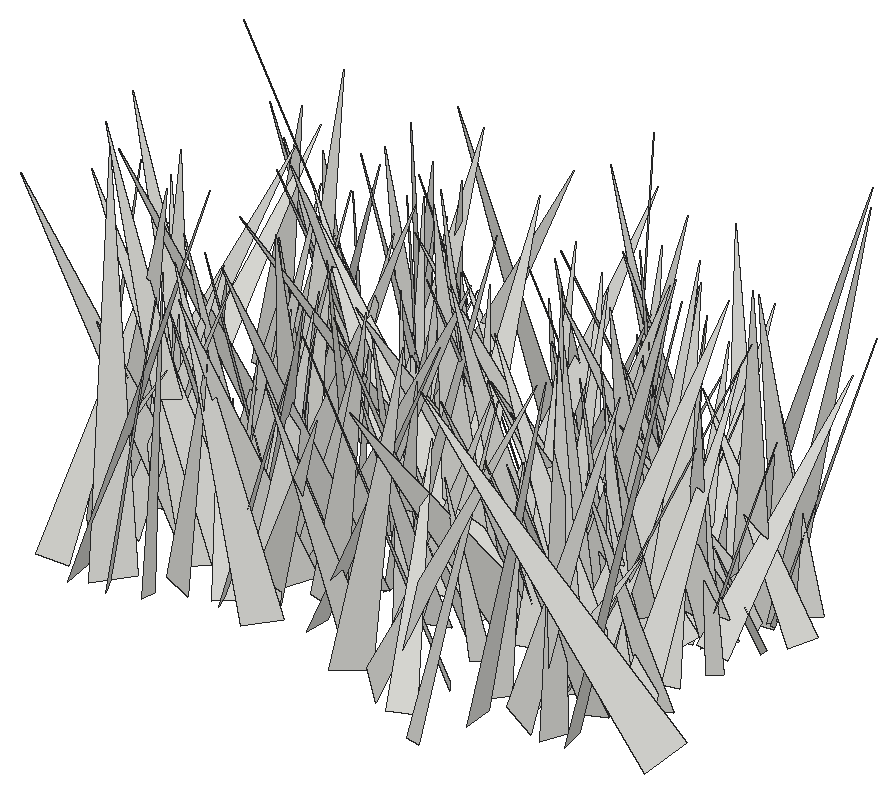
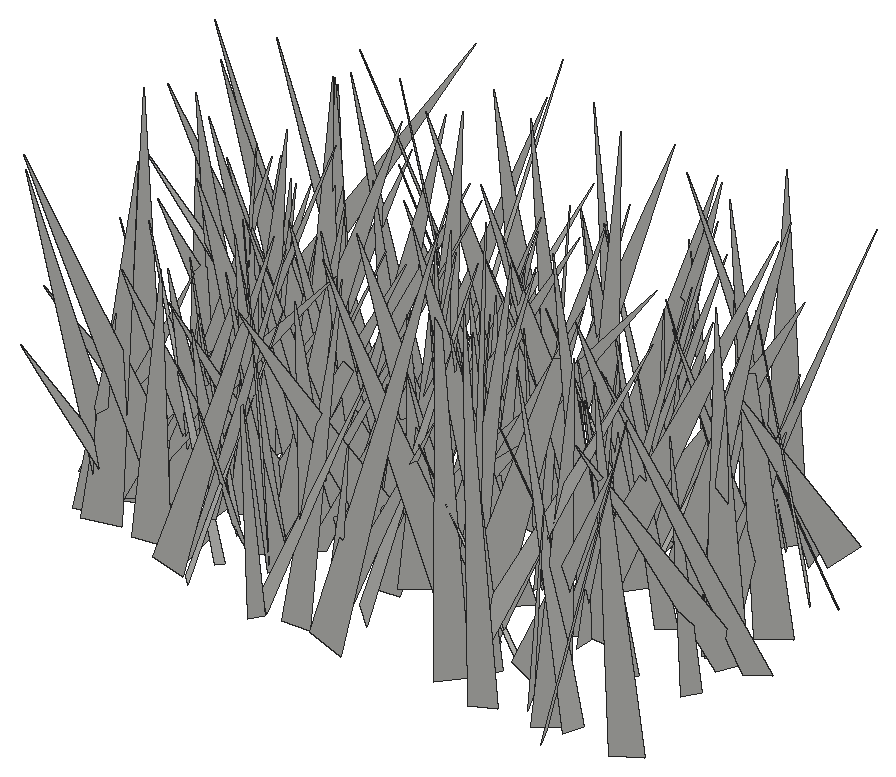
# SketchUp Ruby script. Lengths in inches.
U = 1.inch
M = Sketchup.active_model
def pt(a) = Geom::Point3d.new(a.map { |v| v * U })
def face(e, loops, mat)
  f = e.add_face(loops[0].map { |a| pt(a) })
  loops[1..].each { |l| e.add_face(l.map { |a| pt(a) }).erase! }
  f.material = f.back_material = mat if mat
  f
end
# faces: each face lists its corners as indices into pts; further lists are holes
def faces(e, pts, list, mat = nil) = list.each { |f| face(e, (f[0].is_a?(Array) ? f : [f]).map { |l| l.map { |i| pts[i] } }, mat) }
# xy, xz, yz: faces in a plane at the given z, y or x. An outline is a flat list of corners, or four numbers for a rectangle; further outlines are holes
def ring(l) = l.size == 4 ? [[l[0], l[1]], [l[2], l[1]], [l[2], l[3]], [l[0], l[3]]] : l.each_slice(2).to_a
def flat(e, list, mat, &to3) = list.each { |f| face(e, (f[0].is_a?(Array) ? f : [f]).map { |l| ring(l).map { |u, v| to3.(u, v) } }, mat) }
def xy(e, z, list, mat = nil) = flat(e, list, mat) { |x, y| [x, y, z] }
def xz(e, y, list, mat = nil) = flat(e, list, mat) { |x, z| [x, y, z] }
def yz(e, x, list, mat = nil) = flat(e, list, mat) { |y, z| [x, y, z] }
def lines(e, pts, list) = list.each { |a, b| e.add_line(pt(pts[a]), pt(pts[b])) }
# prism: a flat outline (further loops are holes) pulled along v
def prism(e, loops, v, mat = nil)
  f = face(e, loops, mat); d = Geom::Vector3d.new(v.map { |x| x * U })
  f.pushpull(f.normal.samedirection?(d) ? d.length : -d.length)
end
def box(e, o, s, mat = nil) = prism(e, [[o, [o[0] + s[0], o[1], o[2]], [o[0] + s[0], o[1] + s[1], o[2]], [o[0], o[1] + s[1], o[2]]]], [0, 0, s[2]], mat)
def at(x, y, z, deg = 0) = Geom::Transformation.translation(pt([x, y, z])) * Geom::Transformation.rotation(ORIGIN, Z_AXIS, deg.degrees)
def axes(o, x, y, z) = Geom::Transformation.new([*x, 0, *y, 0, *z, 0, *pt(o).to_a, 1])
def part(name) = M.definitions.add(name)
# library, detail: a bought-in or finely detailed component or shape, given as its bounding box
def library(name, o, s) = part(name).tap { |d| box(d.entities, o, s) }
def detail(e, o, s) = box(e.add_group.entities, o, s)
def put(e, d, t, mat = nil) = e.add_instance(d, t).tap { |i| i.material = mat if mat }
def group(e, t, mat = nil) = e.add_group.tap { |g| g.transformation = t; g.material = mat if mat }.entities
root = M.entities
c1 = part("fur_instance\#9")
p = [[0.8125,0,1.79],[0.67,-0.02,1.48],[0,-0.11,0],[0,0.11,0]]
faces(c1.entities,p,[[0,1,2,3]])
put(root,c1,axes([521.01,81.8,-21.66],[3.09687,5.17866,0.3937],[4.90573,-3.06729,1.75775],[-1.70508,0.58082,5.7723]))
put(root,c1,axes([528.17,86.52,-21.86],[-7.44265,2.94787,0.75024],[2.95668,6.54484,3.6151],[-0.71474,-3.62229,7.14241]))
put(root,c1,axes([516.07,84.62,-21.86],[5.12868,-4.19399,1.94705],[-4.5125,-5.17419,0.74098],[-1.00889,1.82269,6.58361]))
put(root,c1,axes([517.27,84.22,-21.86],[5.08074,5.57509,0.64514],[5.46993,-4.72427,-2.25231],[1.25607,-1.97773,7.19879]))
put(root,c1,axes([511.91,85.02,-21.66],[2.26565,-5.57265,3.25786],[-5.77256,-3.29433,-1.62055],[-2.88887,2.21229,5.79322]))
put(root,c1,axes([507.94,85.42,-21.86],[-0.80392,-5.00028,1.94874],[-5.12712,1.2977,1.21465],[1.58527,1.66129,4.91668]))
put(root,c1,axes([506.07,84.01,-21.86],[4.42151,2.80893,1.55928],[2.73673,-4.68252,0.67492],[-1.68278,-0.23477,5.19464]))
put(root,c1,axes([519.25,83.37,-21.86],[-2.44616,4.11048,0.29857],[4.09909,2.46258,-0.31948],[0.42742,-0.0923,4.7726]))
put(root,c1,axes([511,86.26,-21.66],[2.55159,-4.81811,0.15811],[-4.66384,-2.42197,1.46026],[1.21971,0.81832,5.25284]))
put(root,c1,axes([505.93,84.46,-21.86],[5.91163,-3.56463,4.13587],[-4.286,-6.80601,0.26026],[-3.38262,2.39395,6.89828]))
put(root,c1,axes([514.3125,86.87,-21.86],[-5.24413,-0.63684,1.6828],[-0.10679,5.28634,1.66778],[1.7961,-1.54509,5.01248]))
put(root,c1,axes([519.61,85.54,-21.66],[-5.18196,-4.15409,0.26027],[-4.02731,4.89921,-1.98883],[-1.05116,1.70828,6.3367]))
put(root,c1,axes([521.53,84.66,-21.86],[6.35559,1.23086,1.81432],[1.1106,-6.60444,0.5901],[-1.89033,0.25813,6.44673]))
put(root,c1,axes([504.71,84.05,-21.86],[7.43833,2.19546,1.23858],[2.06036,-7.51855,0.95355],[-1.45225,0.57818,7.69672]))
put(root,c1,axes([511.29,86.12,-21.86],[-2.70694,-4.99144,1.16007],[-5.08628,2.45713,-1.29614],[-0.62448,1.62351,5.52829]))
put(root,c1,axes([507.77,84.05,-21.66],[-5.27031,-0.93158,1.82448],[-1.52104,5.15288,-1.7627],[1.37223,2.13373,5.05341]))
put(root,c1,axes([511.16,87.9,-21.66],[3.93068,-5.30389,1.53813],[-4.85639,-4.21869,-2.1367],[-2.62918,-0.13704,6.24628]))
put(root,c1,axes([509.61,85.91,-21.86],[5.27684,1.71083,0.85913],[1.8324,-5.24307,-0.81398],[-0.55438,-1.04563,5.4872]))
put(root,c1,axes([510.93,86.66,-21.86],[-4.07714,-4.72232,1.18622],[-4.85623,4.056,-0.54439],[0.3528,1.25658,6.21506]))
put(root,c1,axes([522.71,85.41,-21.86],[2.74298,6.25055,1.8619],[6.47418,-2.36552,-1.59662],[0.78801,-2.32269,6.63657]))
put(root,c1,axes([524.76,87.02,-21.66],[-0.6126,-5.21006,0.97224],[-5.10965,0.32064,-1.50131],[-1.40764,1.1035,5.02654]))
put(root,c1,axes([517.81,88.86,-21.66],[-5.57338,-5.53642,0.81265],[-5.27737,5.58191,1.83481],[1.86058,-0.75178,7.63858]))
put(root,c1,axes([509.39,86.82,-21.86],[-1.65671,-3.63214,1.3485],[-3.6613,1.94738,0.7471],[1.26719,0.87797,3.92161]))
put(root,c1,axes([521.15,86.21,-21.86],[-3.54773,2.23846,2.32232],[2.39169,4.14191,-0.33862],[2.16418,-0.90784,4.1812]))
put(root,c1,axes([518.2,90.875,-21.86],[6.60243,-3.6292,1.16999],[-2.40466,-5.77841,-4.35427],[-2.95933,-3.40161,6.14845]))
put(root,c1,axes([511.16,85.8,-21.86],[3.9195,-3.82723,2.46639],[-4.43668,-3.94163,0.93419],[-1.02305,2.43088,5.39791]))
put(root,c1,axes([512.7,87.59,-21.86],[0.32033,-6.88611,1.90206],[-6.92731,0.16595,1.76741],[1.74605,1.92169,6.66313]))
put(root,c1,axes([501.88,86.5625,-21.86],[3.27011,3.05252,0.13659],[2.8317,-2.95233,-1.81533],[1.14804,-1.41282,4.08853]))
put(root,c1,axes([509.76,85.68,-21.86],[-2.46678,3.0111,0.36551],[3.02886,2.4705,0.08915],[0.1623,-0.33942,3.8915]))
put(root,c1,axes([508.62,89.48,-21.66],[8.12463,-0.31909,0.21051],[-0.21684,-7.53553,-3.0536],[-0.31483,-3.04462,7.53571]))
put(root,c1,axes([513.31,89.12,-21.66],[0.28426,-7.43419,0.75555],[-7.30944,-0.43371,-1.51752],[-1.55247,0.68085,7.28321]))
put(root,c1,axes([510.72,87.36,-21.86],[-2.89225,-3.68575,0.79235],[-3.76683,2.78458,-0.79678],[-0.15371,1.11313,4.61682]))
put(root,c1,axes([505.41,89.15,-21.86],[-7.55604,-1.18176,1.01335],[-0.88861,7.39753,2.00103],[1.27821,-1.84315,7.38147]))
put(root,c1,axes([516.8125,85.96,-21.86],[4.76351,-2.22786,1.63166],[-2.67424,-4.53288,1.61806],[-0.68857,2.19233,5.00362]))
put(root,c1,axes([524.37,85.24,-21.86],[-7.61718,0.0241,1.98426],[-0.51537,7.57673,-2.07045],[1.91631,2.1335,7.33043]))
put(root,c1,axes([513.29,86.28,-21.86],[6.06997,0.80019,0.53139],[0.73411,-6.05703,0.73529],[-0.61948,0.66277,6.07817]))
put(root,c1,axes([519.12,87.84,-21.86],[1.11597,-3.30458,1.27259],[-3.40234,-1.37051,-0.57526],[-0.98175,0.99326,3.44016]))
put(root,c1,axes([507.96,86.89,-21.66],[-2.53782,7.33959,2.16761],[7.45924,1.86167,2.42953],[-1.71111,-2.77006,7.37615]))
put(root,c1,axes([503.67,83.97,-21.66],[-4.95607,3.58078,0.35964],[3.00453,4.45388,-2.94106],[1.98095,2.2034,5.36049]))
put(root,c1,axes([509.98,86.38,-21.66],[-2.8355,7.09509,0.7949],[6.33308,2.10473,3.80453],[-3.2961,-2.05963,6.62616]))
put(root,c1,axes([522.11,86.8,-21.86],[0.48143,3.7055,0.846],[3.27794,0.02687,-1.98307],[1.92393,-0.97302,3.16701]))
put(root,c1,axes([516.48,88.82,-21.86],[0.3349,-5.08877,0.86463],[-5.08924,-0.4702,-0.79617],[-0.86188,0.79915,5.03725]))
put(root,c1,axes([524.95,85.5,-21.86],[7.20277,3.49638,1.97973],[3.12762,-7.42996,1.74287],[-2.5223,0.77133,7.81454]))
put(root,c1,axes([522.8125,87.74,-21.86],[4.6761,-4.10232,2.76945],[-4.45315,-5.14998,-0.1096],[-2.16064,1.73593,6.21956]))
put(root,c1,axes([509.41,86.43,-21.86],[1.88548,3.67223,0.79609],[3.49899,-2.04056,1.12569],[-1.36969,-0.15771,3.97154]))
put(root,c1,axes([509.57,90.0625,-21.86],[7.0973,-2.99001,1.53723],[-2.6894,-7.20395,-1.59536],[-2.01752,-0.91535,7.53436]))
put(root,c1,axes([524.17,88.44,-21.86],[-5.92654,3.46188,1.28835],[3.68281,5.72588,1.55549],[0.28525,-1.99951,6.68498]))
put(root,c1,axes([526.1,88.89,-21.86],[0.22156,-4.52657,1.23949],[-4.53883,-0.5223,-1.09609],[-1.19379,1.1457,4.39744]))
put(root,c1,axes([502.24,89.59,-21.86],[1.15039,-7.47242,1.55869],[-7.41634,-0.72104,2.01691],[1.80677,1.79806,7.28646]))
put(root,c1,axes([508.58,88.03,-21.86],[-4.07706,-2.14403,0.24298],[-2.12817,3.90987,-1.20919],[-0.35608,1.18084,4.44491]))
put(root,c1,axes([503.11,86.625,-21.66],[4.45887,4.52554,1.75159],[4.30275,-4.78695,1.41478],[-2.24387,-0.18639,6.19358]))
put(root,c1,axes([504.19,87.36,-21.86],[0.82135,5.31818,1.14764],[5.3338,-0.55827,-1.23031],[1.07271,-1.29616,5.2387]))
put(root,c1,axes([503.71,88.63,-21.66],[4.52674,3.32324,0.78926],[3.39525,-4.2348,-1.64226],[0.37301,-1.78348,5.37013]))
put(root,c1,axes([503.77,90.49,-21.86],[1.96703,-4.29578,0.10046],[-4.18734,-1.94112,-1.01553],[-0.96439,-0.33368,4.61429]))
put(root,c1,axes([511.44,88.99,-21.86],[5.85705,-5.48153,0.51052],[-5.36351,-5.5136,2.33363],[1.24121,2.04104,7.67505]))
put(root,c1,axes([521.9,89.69,-21.86],[-4.92901,3.2655,3.81824],[4.17297,5.6397,0.56365],[2.798,-2.65855,5.88565]))
put(root,c1,axes([509.59,88.1,-21.86],[-2.16703,-5.16397,2.37315],[-5.48971,1.24499,-2.30381],[-1.47021,2.96275,5.10441]))
put(root,c1,axes([519.07,91.24,-21.66],[-5.21619,-2.22313,1.39253],[-1.54183,5.10575,2.37575],[2.12232,-1.75473,5.14847]))
put(root,c1,axes([504.39,89.39,-21.86],[2.0816,-3.74764,1.04429],[-3.88491,-2.06538,0.3318],[-0.20701,1.076,4.27408]))
put(root,c1,axes([509.35,89.49,-21.86],[2.82941,3.82153,3.56935],[4.50896,-3.83832,0.53527],[-2.64833,-2.45217,4.72474]))
put(root,c1,axes([513.73,90.11,-21.86],[4.68677,-2.0034,0.66372],[-1.95488,-4.73014,-0.47351],[-0.79535,-0.17932,5.07496]))
put(root,c1,axes([519.375,90.9,-21.66],[4.80769,-4.80499,2.60276],[-4.52111,-5.44469,-1.70033],[-3.0695,0.49361,6.58109]))
put(root,c1,axes([525.09,89.38,-21.86],[0.28684,-3.45624,1.82339],[-3.70035,-0.82791,-0.9872],[-1.25608,1.64973,3.32465]))
put(root,c1,axes([514.03,89.74,-21.86],[6.05057,5.41917,1.99571],[5.77348,-5.74186,-1.9125],[-0.1309,-2.76104,7.89425]))
put(root,c1,axes([524,91.14,-21.86],[4.64418,-2.47093,1.08294],[-2.19439,-4.71399,-1.3452],[-1.56935,-0.72073,5.0857]))
put(root,c1,axes([519.22,91,-21.86],[-2.4025,-2.92839,0.44923],[-2.80853,2.4353,0.85486],[0.94311,-0.20767,3.69008]))
put(root,c1,axes([515.65,88.11,-21.86],[-5.70107,0.73605,0.76728],[0.48907,5.53142,-1.67238],[0.94409,1.57933,5.49974]))
put(root,c1,axes([521.3,90.39,-21.66],[-4.03956,-5.75099,0.92293],[-5.66396,3.6166,-2.25467],[-1.3584,2.0224,6.65646]))
put(root,c1,axes([513.4,90.83,-21.86],[-1.65824,-4.82946,1.36253],[-4.95542,1.80194,0.35604],[0.78993,1.16588,5.09379]))
put(root,c1,axes([523.46,90.27,-21.86],[-4.23654,2.45749,2.21286],[2.8358,4.54981,0.37637],[1.70124,-1.46429,4.88322]))
put(root,c1,axes([510.73,88.74,-21.86],[6.30569,-0.68619,2.05979],[-1.17683,-6.39727,1.4715],[-1.82446,1.75482,6.16987]))
put(root,c1,axes([508.27,92.13,-21.66],[-1.35129,-7.71927,0.81651],[-7.46816,1.06686,-2.27338],[-2.11671,1.16382,7.49966]))
put(root,c1,axes([513.27,90.72,-21.86],[-1.26744,-3.38882,1.28492],[-3.35573,1.6115,0.94004],[1.36901,0.81271,3.49382]))
put(root,c1,axes([510.46,91.95,-21.66],[5.99792,1.55177,2.60045],[2.40829,-5.94226,-2.00876],[-1.83589,-2.72525,5.86071]))
put(root,c1,axes([521.625,89.21,-21.66],[7.44072,-1.6859,2.03296],[-2.09272,-7.4711,1.46382],[-1.61112,1.91833,7.48758]))
put(root,c1,axes([522.96,88.12,-21.66],[-0.55252,7.61083,1.2014],[7.43516,0.84266,-1.91879],[2.02152,-1.01911,7.38568]))
put(root,c1,axes([522.42,91.25,-21.86],[-4.86082,-0.82699,0.28427],[-0.77768,4.82218,0.73078],[0.39992,-0.67448,4.87621]))
put(root,c1,axes([524.03,89.23,-21.66],[-5.16392,-1.1559,0.80889],[-1.35151,4.93357,-1.57791],[0.40477,1.72635,5.05098]))
put(root,c1,axes([508.83,87.21,-21.86],[-6.46453,1.71895,1.7422],[0.79023,6.12289,-3.109],[2.31637,2.70842,5.92275]))
put(root,c1,axes([523.9,90.1,-21.86],[-3.13424,-4.33981,2.11732],[-4.81159,3.01955,-0.93345],[0.40688,2.2779,5.27125]))
put(root,c1,axes([508,89.85,-21.86],[2.7326,-2.75522,2.01665],[-3.2693,-2.85632,0.52755],[-0.98478,1.83723,3.84448]))
put(root,c1,axes([515.875,91.38,-21.86],[3.74176,-6.61768,2.63887],[-6.89022,-4.11933,-0.5604],[-1.81167,1.99888,7.58159]))
put(root,c1,axes([506.16,89.92,-21.86],[-2.60972,7.0339,1.93347],[7.14895,2.0575,2.16424],[-1.45142,-2.51309,7.18348]))
put(root,c1,axes([517.49,90.99,-21.86],[-6.72983,3.60579,0.05795],[3.45053,6.40273,2.3226],[-1.04828,-2.07339,7.27309]))
put(root,c1,axes([508.75,90.04,-21.66],[6.76451,-3.26106,1.25254],[-3.47694,-6.54929,1.72622],[-0.33809,2.1058,7.30844]))
put(root,c1,axes([522.96,87.76,-21.66],[6.18332,3.30926,0.01495],[3.17233,-5.93637,1.96995],[-0.9422,1.73008,6.73082]))
put(root,c1,axes([503.08,91.77,-21.86],[2.15592,-3.18911,0.31319],[-3.19535,-2.16794,-0.07942],[-0.24138,0.21478,3.84865]))
put(root,c1,axes([505.49,91.33,-21.86],[0.14432,-5.01914,1.5992],[-4.96199,0.40759,1.72702],[1.76858,1.55311,4.71487]))
put(root,c1,axes([509.18,87.98,-21.66],[4.35483,5.04158,0.80125],[4.65214,-4.35304,2.10539],[-2.1017,0.81089,6.32055]))
put(root,c1,axes([522.05,87.8125,-21.86],[1.21236,6.8418,0.01969],[6.58716,-1.17263,1.87473],[-1.84929,0.30844,6.6907]))
put(root,c1,axes([525.7,87.86,-21.66],[-4.59878,4.14257,0.47856],[3.69105,4.37512,-2.40275],[1.94062,1.49539,5.70408]))
put(root,c1,axes([508.4,90.45,-21.86],[4.45017,0.43948,1.54669],[0.28501,-4.6951,0.51402],[-1.58245,0.39027,4.44218]))
put(root,c1,axes([504.89,89.44,-21.86],[-0.8171,5.77252,0.59098],[5.63961,0.64951,1.4532],[-1.36602,-0.77139,5.64605]))
put(root,c1,axes([516.68,92.74,-21.86],[3.47774,-1.50181,0.39234],[-1.2719,-3.30895,-1.39185],[-0.88975,-1.13996,3.5232]))
put(root,c1,axes([502.6875,91.61,-21.86],[3.75494,-4.9741,2.2471],[-5.32599,-3.93562,0.18806],[-1.1937,1.91308,6.22943]))
put(root,c1,axes([510.8125,91.56,-21.86],[2.85129,3.39796,1.84964],[3.79237,-2.9092,-0.50161],[-0.76499,-1.75715,4.40731]))
put(root,c1,axes([524.74,90.33,-21.86],[-2.30774,6.81626,2.09214],[7.04491,2.51871,-0.43516],[1.09893,-1.8327,7.18315]))
put(root,c1,axes([515.68,93.22,-21.86],[-2.19661,-7.3796,0.4517],[-6.30745,1.62463,-4.13089],[-3.85727,1.54587,6.49764]))
put(root,c1,axes([514.49,95.29,-21.86],[6.08199,-2.63161,2.26399],[-1.13407,-5.82276,-3.72169],[-3.281,-2.8656,5.48316]))
put(root,c1,axes([511.36,92.77,-21.86],[4.77577,-2.2799,0.31782],[-2.26651,-4.78515,-0.26858],[-0.40236,-0.10607,5.28524]))
put(root,c1,axes([514.18,91.1,-21.66],[-4.44973,5.42889,0.1833],[5.21151,4.19987,2.12315],[-1.53186,-1.48148,6.69068]))
put(root,c1,axes([524.9,93.57,-21.66],[2.07945,-5.56592,1.40736],[-5.43571,-2.39045,-1.42237],[-1.84751,0.76846,5.76892]))
put(root,c1,axes([520.09,89.32,-21.66],[0.51601,7.02264,0.2402],[6.84431,-0.55684,1.57697],[-1.5908,-0.11784,6.86272]))
put(root,c1,axes([507.3,92.39,-21.86],[2.93725,2.51058,1.33666],[2.80043,-2.8887,-0.72813],[-0.49727,-1.43859,3.79478]))
put(root,c1,axes([523.35,93.94,-21.86],[2.32461,-5.72045,0.33614],[-5.68592,-2.25756,0.90225],[0.71192,0.64824,6.10846]))
put(root,c1,axes([520.72,94.3125,-21.86],[0.56796,-5.36738,0.34113],[-5.01782,-0.65229,-1.90884],[-1.93561,0.11605,5.04853]))
put(root,c1,axes([524.51,89.02,-21.66],[-6.77077,3.15469,0.89527],[2.64884,6.47215,-2.77341],[1.93319,2.18084,6.93567]))
put(root,c1,axes([523.82,93.07,-21.86],[-4.01783,2.35497,0.3103],[2.27352,3.63609,1.84258],[-0.68795,-1.73727,4.27712]))
put(root,c1,axes([521.38,93.99,-21.86],[2.40943,-6.40182,1.38295],[-6.51779,-2.4885,-0.16399],[-0.64358,1.23501,6.83826]))
put(root,c1,axes([519.46,94.28,-21.86],[0.8568,-5.86099,0.80486],[-5.91149,-0.87995,-0.11477],[-0.231,0.77949,5.92218]))
put(root,c1,axes([513.79,93.8,-21.86],[1.49133,-6.04191,1.54576],[-6.23212,-1.50337,0.13646],[-0.23383,1.53405,6.22175]))
put(root,c1,axes([516.67,91.53,-21.66],[-7.00273,-0.39667,0.95685],[-0.59042,6.90153,-1.45992],[0.85107,1.52402,6.86034]))
put(root,c1,axes([519.11,94.78,-21.86],[-7.35388,-1.92649,0.06127],[-1.88282,7.23164,1.39751],[0.41243,-1.33667,7.47248]))
put(root,c1,axes([515.4,90.57,-21.86],[-3.83392,6.10516,1.11787],[5.9137,3.99214,-1.52073],[1.88436,-0.10697,7.04694]))
put(root,c1,axes([507.01,93.84,-21.86],[-4.71927,-1.33587,1.95814],[-1.09743,5.09822,0.83318],[2.10107,-0.33763,4.83341]))
put(root,c1,axes([515.02,94.55,-21.86],[2.32528,-3.90872,0.2043],[-3.90658,-2.33236,-0.15975],[-0.24182,0.09371,4.54527]))
put(root,c1,axes([523.02,95.65,-21.86],[-7.04471,-1.4589,1.32068],[-0.96261,6.83613,2.41686],[1.71638,-2.15394,6.77607]))
put(root,c1,axes([522.68,91.78,-21.86],[-5.01766,-1.40088,1.70753],[-1.93126,4.83928,-1.7049],[1.07162,2.16194,4.92267]))
put(root,c1,axes([502.01,94.33,-21.86],[4.41728,-0.60705,0.29796],[-0.51929,-4.30631,-1.07505],[-0.43316,-1.02804,4.32726]))
put(root,c1,axes([513.29,90.84,-21.86],[-5.97598,0.81352,1.54005],[0.17172,5.75229,-2.37225],[1.73323,2.235,5.54496]))
put(root,c1,axes([513.79,94.4,-21.86],[4.45698,-3.93649,1.376],[-3.92382,-4.64074,-0.56675],[-1.41173,0.47074,5.91941]))
put(root,c1,axes([520.14,91.86,-21.86],[7.25129,-2.23194,2.73946],[-2.93898,-7.28136,1.84704],[-1.96177,2.6585,7.35875]))
put(root,c1,axes([513.12,93.56,-21.86],[4.15437,2.45212,1.76514],[2.75663,-4.30471,-0.50784],[-1.23677,-1.35794,4.79727]))
put(root,c1,axes([518.11,93.12,-21.86],[3.27115,-5.93629,2.22387],[-6.24966,-2.60094,2.25],[1.06155,2.98013,6.39355]))
put(root,c1,axes([525,95.82,-21.66],[-5.02387,-1.18033,0.42976],[-0.88594,4.58548,2.23734],[0.8905,-2.09699,4.65046]))
put(root,c1,axes([510.04,96.3,-21.86],[3.07442,-7.15508,0.96712],[-6.88437,-3.22185,-1.95131],[-2.1762,0.08396,7.5392]))
put(root,c1,axes([514.88,92.93,-21.86],[-0.37436,4.96388,1.61425],[5.21969,0.34743,0.14211],[-0.02763,-1.62026,4.97594]))
put(root,c1,axes([524.13,93.74,-21.86],[4.65437,1.55789,0.49043],[1.62302,-4.57734,-0.86283],[-0.1826,-0.97553,4.83174]))
put(root,c1,axes([522.78,93.57,-21.86],[3.92843,5.06138,3.38638],[5.5366,-4.64662,0.52215],[-2.53598,-2.30413,6.38572]))
put(root,c1,axes([500.89,92.14,-21.66],[0.65701,6.39206,0.99008],[6.12037,-0.29236,-2.17392],[2.09278,-1.15171,6.04683]))
put(root,c1,axes([512.69,92.08,-21.86],[0.64289,6.12986,1.03372],[6.0316,-0.86662,1.38779],[-1.50455,-0.85491,6.00521]))
put(root,c1,axes([525.89,92.02,-21.86],[-4.92435,-0.05312,0.24709],[-0.15186,4.47527,-2.06445],[0.20202,2.06935,4.47102]))
put(root,c1,axes([511.75,93.99,-21.86],[4.16125,-1.09144,0.28201],[-1.11074,-4.15389,0.31328],[-0.19241,0.37504,4.29058]))
put(root,c1,axes([504.54,94.69,-21.86],[0.76926,-4.66703,1.07076],[-4.59745,-0.41678,1.48633],[1.33832,1.25083,4.49041]))
put(root,c1,axes([518.1,94.53,-21.86],[-4.18794,0.93567,0.33129],[0.9893,4.05153,1.06324],[0.08071,-1.11073,4.15738]))
put(root,c1,axes([513.05,94.24,-21.66],[-3.81075,-5.76969,1.72606],[-6.01138,3.52106,-1.50194],[-0.36316,2.25903,6.74947]))
put(root,c1,axes([516.71,93.71,-21.86],[6.16079,-1.33707,0.34037],[-1.37023,-6.11166,0.79308],[-0.16154,0.84778,6.25413]))
put(root,c1,axes([524.05,94.99,-21.86],[-1.08629,-5.09453,1.21583],[-5.17343,0.84989,-1.06105],[-0.81738,1.39139,5.09985]))
put(root,c1,axes([507.74,93.73,-21.86],[-3.05082,2.35934,0.28628],[2.37608,3.01778,0.45074],[-0.05159,-0.53147,3.83025]))
put(root,c1,axes([506.73,93.41,-21.86],[0.76042,7.54721,2.45249],[7.93568,-0.724,-0.23253],[-0.00259,-2.46349,7.58186]))
put(root,c1,axes([511.79,94.08,-21.86],[4.32475,3.25099,2.86901],[3.37923,-5.06616,0.64681],[-2.71679,-1.12634,5.37159]))
put(root,c1,axes([507.6,92.8,-21.86],[2.99735,3.72962,0.28981],[3.68324,-3.00724,0.60693],[-0.65404,0.15682,4.74613]))
put(root,c1,axes([524.63,95.58,-21.86],[2.16747,-6.96935,1.82134],[-7.20329,-2.08612,0.58967],[0.04123,1.91397,7.27476]))
put(root,c1,axes([523.43,92.77,-21.86],[2.56304,5.03632,1.18387],[4.82189,-2.80423,1.49027],[-1.87495,-0.32715,5.45094]))
put(root,c1,axes([510.53,93.34,-21.86],[-2.56408,6.91655,2.55207],[6.94878,3.17004,-1.60986],[2.46298,-1.74312,7.19872]))
put(root,c1,axes([519.9,93.07,-21.66],[4.92859,0.75105,0.39032],[0.57555,-4.66461,1.7081],[-0.62062,1.63853,4.68375]))
put(root,c1,axes([526.23,94.25,-21.86],[-5.38862,-5.55187,0.24968],[-4.68183,4.34761,-4.37054],[-2.99434,3.19341,6.38427]))
put(root,c1,axes([510.85,95.625,-21.86],[-6.63003,0.58928,2.6026],[0.94805,7.03587,0.82207],[2.49439,-1.10786,6.6052]))
put(root,c1,axes([527.08,95.31,-21.66],[-3.88127,2.88585,0.74535],[2.95869,3.58243,1.53633],[-0.36036,-1.66913,4.58608]))
put(root,c1,axes([523.39,93.67,-21.86],[-4.05743,3.11883,1.27429],[2.94276,4.25195,-1.03673],[1.64046,0.08657,5.0115]))
put(root,c1,axes([502.08,91.88,-21.86],[-2.9172,5.75801,0.16061],[5.28877,2.74872,-2.48273],[2.2824,0.99014,5.95825]))
put(root,c1,axes([518.5625,93.84,-21.86],[-2.91757,4.706,0.99504],[4.75363,2.9987,-0.24403],[0.73452,-0.71423,5.53165]))
put(root,c1,axes([521.0625,94.99,-21.86],[3.30079,2.00098,0.99665],[2.11543,-3.37049,-0.23912],[-0.72261,-0.72685,3.85253]))
put(root,c1,axes([509.43,96.33,-21.66],[-2.97,-5.19915,0.68344],[-5.09037,2.66981,-1.8109],[-1.25951,1.46972,5.70725]))
put(root,c1,axes([514.07,96.98,-21.86],[-4.79453,-5.10071,1.01007],[-5.15614,4.84133,-0.02673],[0.67211,0.75447,7.00029]))
put(root,c1,axes([520.09,97.24,-21.86],[5.66121,2.03663,0.41958],[1.99596,-4.98096,-2.75306],[0.58316,-2.72311,5.34956]))
put(root,c1,axes([525.1,92.87,-21.66],[-2.44099,4.81015,0.04297],[4.37742,2.2412,-2.21652],[1.99437,0.96814,4.91762]))
put(root,c1,axes([523.29,93.04,-21.86],[-3.49002,4.97532,0.38419],[4.70613,3.43753,-1.76559],[1.65943,0.71499,5.81522]))
put(root,c1,axes([508.85,97.6,-21.86],[-4.19902,-6.23031,2.61813],[-6.01537,4.8505,1.89504],[3.08005,0.97931,7.27031]))
put(root,c1,axes([519.15,95.75,-21.86],[-1.46748,5.77462,2.34569],[6.13429,1.76496,-0.50731],[1.10405,-2.13089,5.93652]))
put(root,c1,axes([518.46,96.09,-21.86],[5.41159,0.09186,1.28906],[0.07062,-5.56242,0.09991],[-1.29039,0.08081,5.41145]))
put(root,c1,axes([521.98,94.87,-21.66],[-4.57761,1.25738,1.06742],[0.91701,4.55759,-1.43608],[1.37093,1.14988,4.52473]))
put(root,c1,axes([525.02,97.47,-21.86],[2.11565,-6.08651,1.80009],[-6.2822,-2.27872,-0.32139],[-0.90548,1.58863,6.43571]))
put(root,c1,axes([515.68,92.88,-21.66],[-5.17652,4.83446,1.05401],[3.91261,4.93311,-3.41105],[3.02894,1.88989,6.20751]))
put(root,c1,axes([508.23,97.54,-21.86],[5.48101,-1.25937,0.85366],[-1.15676,-5.52263,-0.72019],[-0.98826,-0.52035,5.57753]))
put(root,c1,axes([508.77,98.82,-21.66],[7.2919,-1.58164,0.56037],[-1.39543,-7.10365,-1.89164],[-0.93186,-1.73896,7.21769]))
put(root,c1,axes([508.07,96.11,-21.86],[3.45283,2.51437,0.03768],[2.48973,-3.40925,-0.65094],[0.3531,-0.54815,4.22141]))
put(root,c1,axes([515.14,96.95,-21.86],[-4.21656,2.08304,0.19454],[2.06998,4.09043,1.06765],[-0.30342,-1.04195,4.58024]))
put(root,c1,axes([520.26,98.79,-21.86],[-3.59271,-3.52154,0.36411],[-3.38524,3.56898,1.11534],[1.03633,-0.55007,4.90559]))
put(root,c1,axes([525.92,97.2,-21.86],[1.42768,-3.34431,1.65268],[-3.54003,-1.77266,-0.52903],[-1.17641,1.27565,3.59761]))
put(root,c1,axes([509.28,97.27,-21.66],[-6.03257,-5.76703,0.56772],[-5.59645,5.58532,-2.7307],[-1.50355,2.34912,7.8863]))
put(root,c1,axes([515.41,98.96,-21.86],[-0.67207,-6.04885,0.74296],[-6.03248,0.76649,0.78356],[0.86591,0.6451,6.03542]))
put(root,c1,axes([521.33,98.49,-21.86],[-0.74587,-6.40704,1.23448],[-6.45249,0.53969,-1.09751],[-0.96927,1.33753,6.35625]))
put(root,c1,axes([509.28,96.76,-21.66],[5.54301,-4.89223,1.08245],[-4.92161,-5.01325,2.54471],[0.93987,2.60075,6.94141]))
put(root,c1,axes([504.3125,99.01,-21.86],[4.76035,-4.27512,0.72339],[-4.20428,-4.81383,-0.78223],[-1.06017,-0.10597,6.35025]))
put(root,c1,axes([519.18,95.67,-21.86],[5.31118,5.11176,2.74997],[4.78098,-5.96627,1.85658],[-3.29161,-0.41778,7.13385]))
put(root,c1,axes([507.11,97.03,-21.66],[-0.49335,5.1966,1.87912],[5.02115,-0.36617,2.33091],[-2.30734,-1.90798,4.67065]))
put(root,c1,axes([521.24,96.95,-21.86],[-7.32876,-0.97242,0.83606],[-1.07916,7.29688,-0.97277],[0.69283,1.07947,7.32872]))
put(root,c1,axes([524.16,94.6875,-21.66],[7.79418,1.63756,2.08164],[0.8535,-7.67768,2.8441],[-2.50726,2.47704,7.43922]))
put(root,c1,axes([513.85,99.32,-21.86],[-2.25691,-7.5793,1.44794],[-7.71352,2.17504,-0.63772],[-0.20948,1.56823,7.88243]))
put(root,c1,axes([503.37,99.01,-21.66],[6.27835,0.76334,0.54412],[0.88551,-6.03847,-1.74618],[-0.30762,-1.80294,6.07875]))
put(root,c1,axes([517.26,98.4,-21.86],[-3.55918,-3.90599,0.48478],[-3.91702,3.45103,-0.95229],[-0.38568,0.99656,5.19785]))
put(root,c1,axes([506.75,99.68,-21.66],[-0.2881,-6.79413,1.19024],[-6.52945,0.65262,2.14482],[2.22333,1.03623,6.45314]))
put(root,c1,axes([501.06,98.99,-21.86],[1.26894,-6.32164,1.3833],[-6.3592,-0.957,1.46001],[1.19887,1.6149,6.28026]))
put(root,c1,axes([520.66,95.41,-21.86],[1.86893,4.92203,0.04113],[4.36091,-1.67616,2.42774],[-2.28266,0.8277,4.67176]))
put(root,c1,axes([525.49,96.1,-21.66],[-6.79191,0.51616,3.38033],[-0.49773,7.28774,-2.11287],[3.3831,2.10844,6.47551]))
put(root,c1,axes([516.82,99.34,-21.86],[4.05285,-0.43746,0.41546],[-0.3233,-3.95717,-1.01285],[-0.50937,-0.96903,3.94856]))
put(root,c1,axes([514.49,98.22,-21.86],[0.90627,3.33198,1.59944],[3.57947,-1.20149,0.47479],[-0.9207,-1.39138,3.42023]))
put(root,c1,axes([504.07,99.75,-21.86],[-5.14482,-3.13912,1.24988],[-3.04737,5.29445,0.7535],[1.4594,-0.01101,5.97959]))
put(root,c1,axes([505.93,98.1,-21.86],[-3.72029,-1.54775,1.40082],[-1.82397,3.80239,-0.64288],[1.01535,1.15959,3.97778]))
put(root,c1,axes([525.58,95.54,-21.66],[4.27823,3.00126,0.70858],[2.21616,-3.83495,2.86263],[-2.14435,2.02448,4.3722]))
put(root,c1,axes([522.82,97.52,-21.86],[-2.14866,5.91991,1.32548],[6.06222,2.04254,0.70466],[-0.22751,-1.48381,6.25824]))
